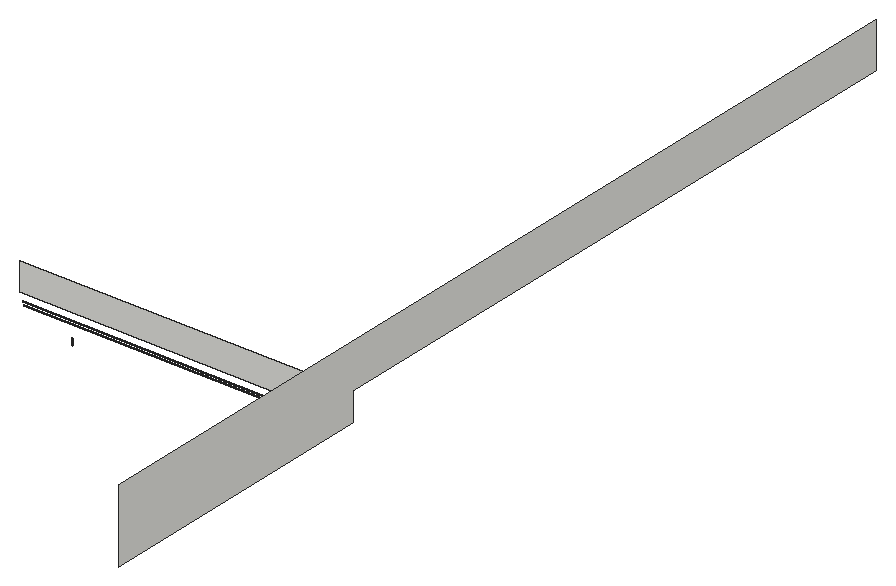
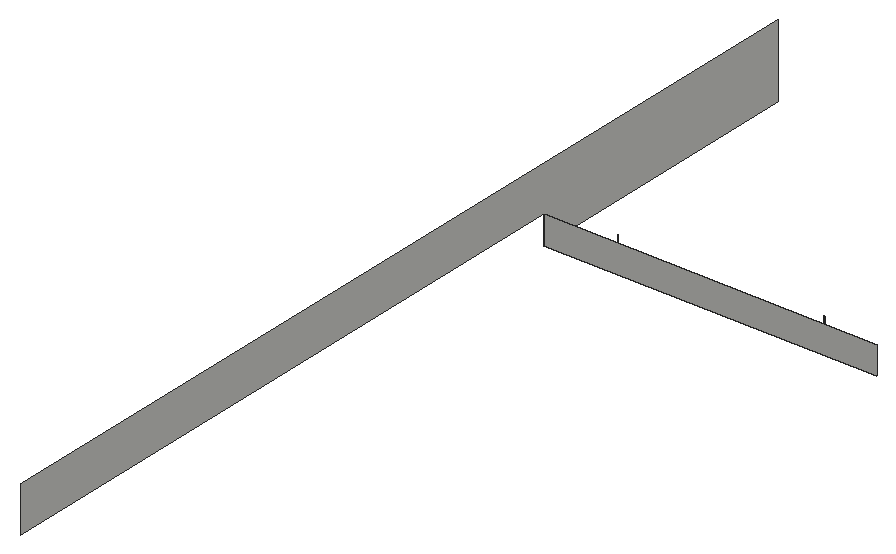
# SketchUp Ruby script. Lengths in inches.
U = 1.inch
M = Sketchup.active_model
def pt(a) = Geom::Point3d.new(a.map { |v| v * U })
def face(e, loops, mat)
  f = e.add_face(loops[0].map { |a| pt(a) })
  loops[1..].each { |l| e.add_face(l.map { |a| pt(a) }).erase! }
  f.material = f.back_material = mat if mat
  f
end
# faces: each face lists its corners as indices into pts; further lists are holes
def faces(e, pts, list, mat = nil) = list.each { |f| face(e, (f[0].is_a?(Array) ? f : [f]).map { |l| l.map { |i| pts[i] } }, mat) }
# xy, xz, yz: faces in a plane at the given z, y or x. An outline is a flat list of corners, or four numbers for a rectangle; further outlines are holes
def ring(l) = l.size == 4 ? [[l[0], l[1]], [l[2], l[1]], [l[2], l[3]], [l[0], l[3]]] : l.each_slice(2).to_a
def flat(e, list, mat, &to3) = list.each { |f| face(e, (f[0].is_a?(Array) ? f : [f]).map { |l| ring(l).map { |u, v| to3.(u, v) } }, mat) }
def xy(e, z, list, mat = nil) = flat(e, list, mat) { |x, y| [x, y, z] }
def xz(e, y, list, mat = nil) = flat(e, list, mat) { |x, z| [x, y, z] }
def yz(e, x, list, mat = nil) = flat(e, list, mat) { |y, z| [x, y, z] }
def lines(e, pts, list) = list.each { |a, b| e.add_line(pt(pts[a]), pt(pts[b])) }
# prism: a flat outline (further loops are holes) pulled along v
def prism(e, loops, v, mat = nil)
  f = face(e, loops, mat); d = Geom::Vector3d.new(v.map { |x| x * U })
  f.pushpull(f.normal.samedirection?(d) ? d.length : -d.length)
end
def box(e, o, s, mat = nil) = prism(e, [[o, [o[0] + s[0], o[1], o[2]], [o[0] + s[0], o[1] + s[1], o[2]], [o[0], o[1] + s[1], o[2]]]], [0, 0, s[2]], mat)
def at(x, y, z, deg = 0) = Geom::Transformation.translation(pt([x, y, z])) * Geom::Transformation.rotation(ORIGIN, Z_AXIS, deg.degrees)
def axes(o, x, y, z) = Geom::Transformation.new([*x, 0, *y, 0, *z, 0, *pt(o).to_a, 1])
def part(name) = M.definitions.add(name)
# library, detail: a bought-in or finely detailed component or shape, given as its bounding box
def library(name, o, s) = part(name).tap { |d| box(d.entities, o, s) }
def detail(e, o, s) = box(e.add_group.entities, o, s)
def put(e, d, t, mat = nil) = e.add_instance(d, t).tap { |i| i.material = mat if mat }
def group(e, t, mat = nil) = e.add_group.tap { |g| g.transformation = t; g.material = mat if mat }.entities
root = M.entities
xz(root,336,[[179,231,340,231.5]])
xz(root,338,[[177,231,342,231.5]])
xz(root,344,[[171,231,348,246]])
yz(root,348,[[188,231,344,231,344,246,692,246,692,270,188,270]])
p = [[326.15,322.09,231],[326.21,322.03,231],[326.21,322.03,234],[326.15,322.09,234],[326.04,322.2,231],[326.1,322.14,231],
  [326.1,322.14,234],[326.04,322.2,234],[325.98,322.25,231],[325.98,322.25,234],[216.32,322.3,231],[216.38,322.25,231],
  [216.38,322.25,234],[216.32,322.3,234],[216.26,322.35,231],[216.26,322.35,234],[216.14,322.45,231],[216.2,322.4,231],
  [216.2,322.4,234],[216.14,322.45,234],[216.07,322.49,231],[216.07,322.49,234],[215.9375,322.58,231],[216.01,322.53,231],
  [216.01,322.53,234],[215.9375,322.58,234],[215.8,322.65,231],[215.87,322.61,231],[215.87,322.61,234],[215.8,322.65,234],
  [215.59,322.75,231],[215.66,322.72,231],[215.66,322.72,234],[215.59,322.75,234],[215.73,322.6875,231],[215.73,322.6875,234],
  [215.3,322.86,231],[215.37,322.84,231],[215.37,322.84,234],[215.3,322.86,234],[215.44,322.8125,231],[215.52,322.78,231],
  [215.52,322.78,234],[215.44,322.8125,234],[215.14,322.91,231],[215.22,322.89,231],[215.22,322.89,234],[215.14,322.91,234],
  [215.07,322.92,231],[215.07,322.92,234]]
faces(root,p,[[0,1,2,3],[4,5,6,7],[5,0,3,6],[8,4,7,9],[10,11,12,13],[14,10,13,15],[16,17,18,19],[20,16,19,21],
  [17,14,15,18],[22,23,24,25],[23,20,21,24],[26,27,28,29],[27,22,25,28],[30,31,32,33],[34,26,29,35],[31,34,35,32],
  [36,37,38,39],[40,41,42,43],[37,40,43,38],[41,30,33,42],[44,45,46,47],[48,44,47,49],[45,36,39,46]])
